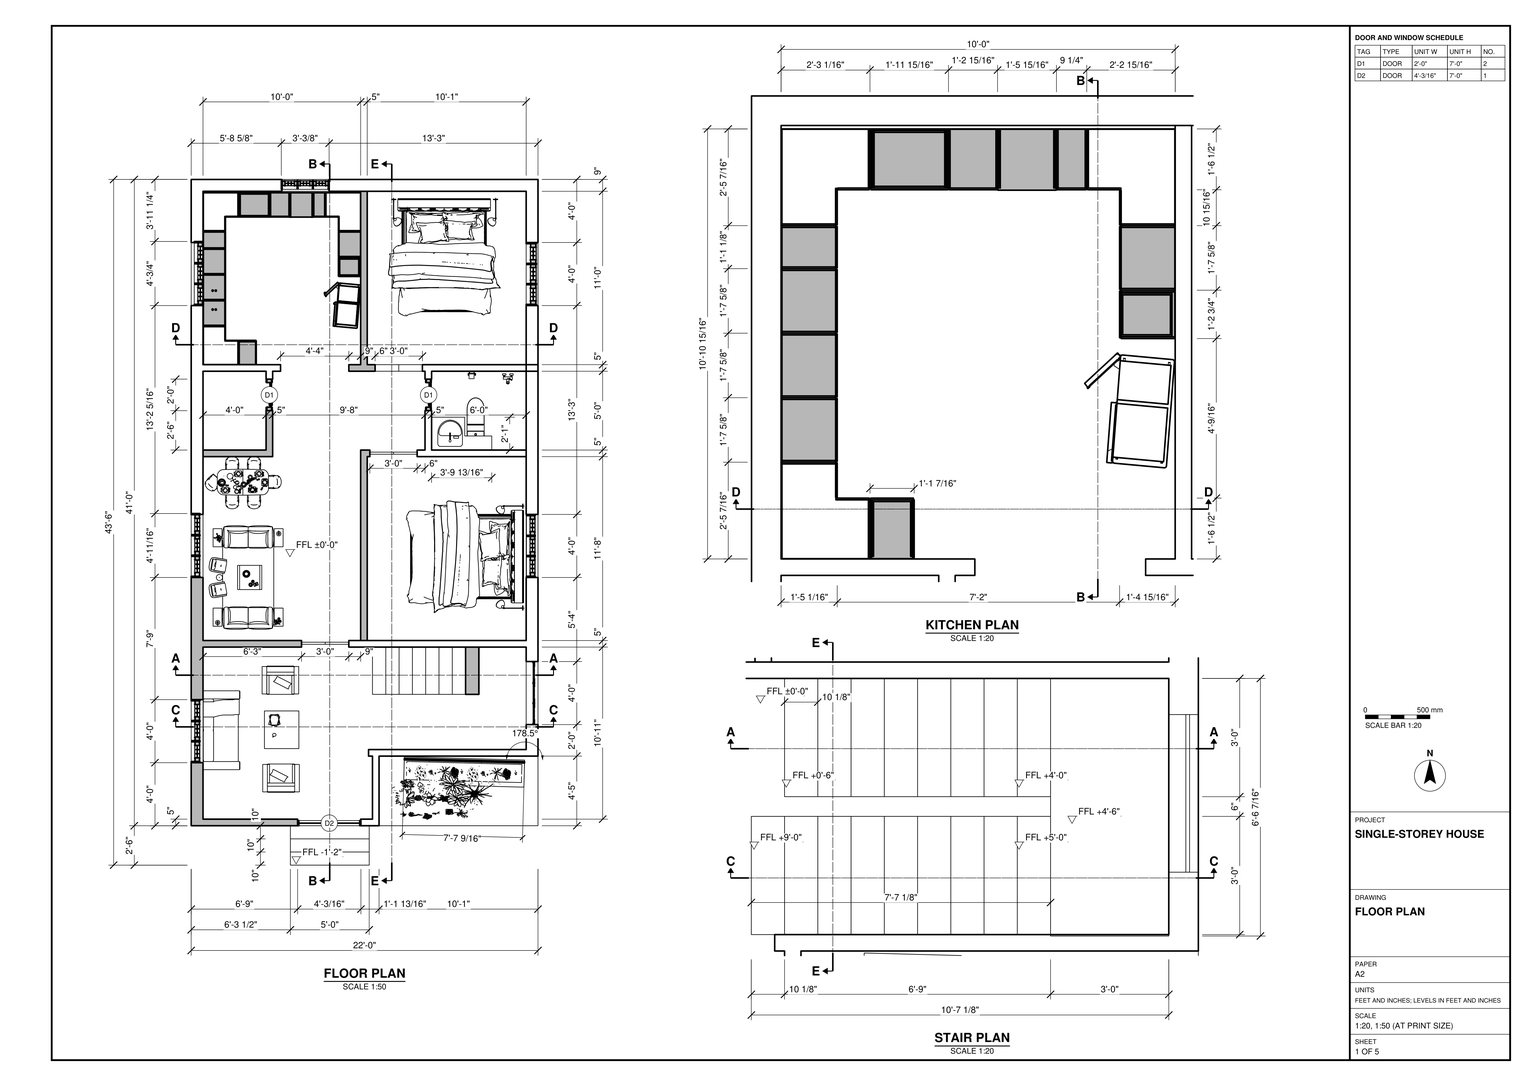
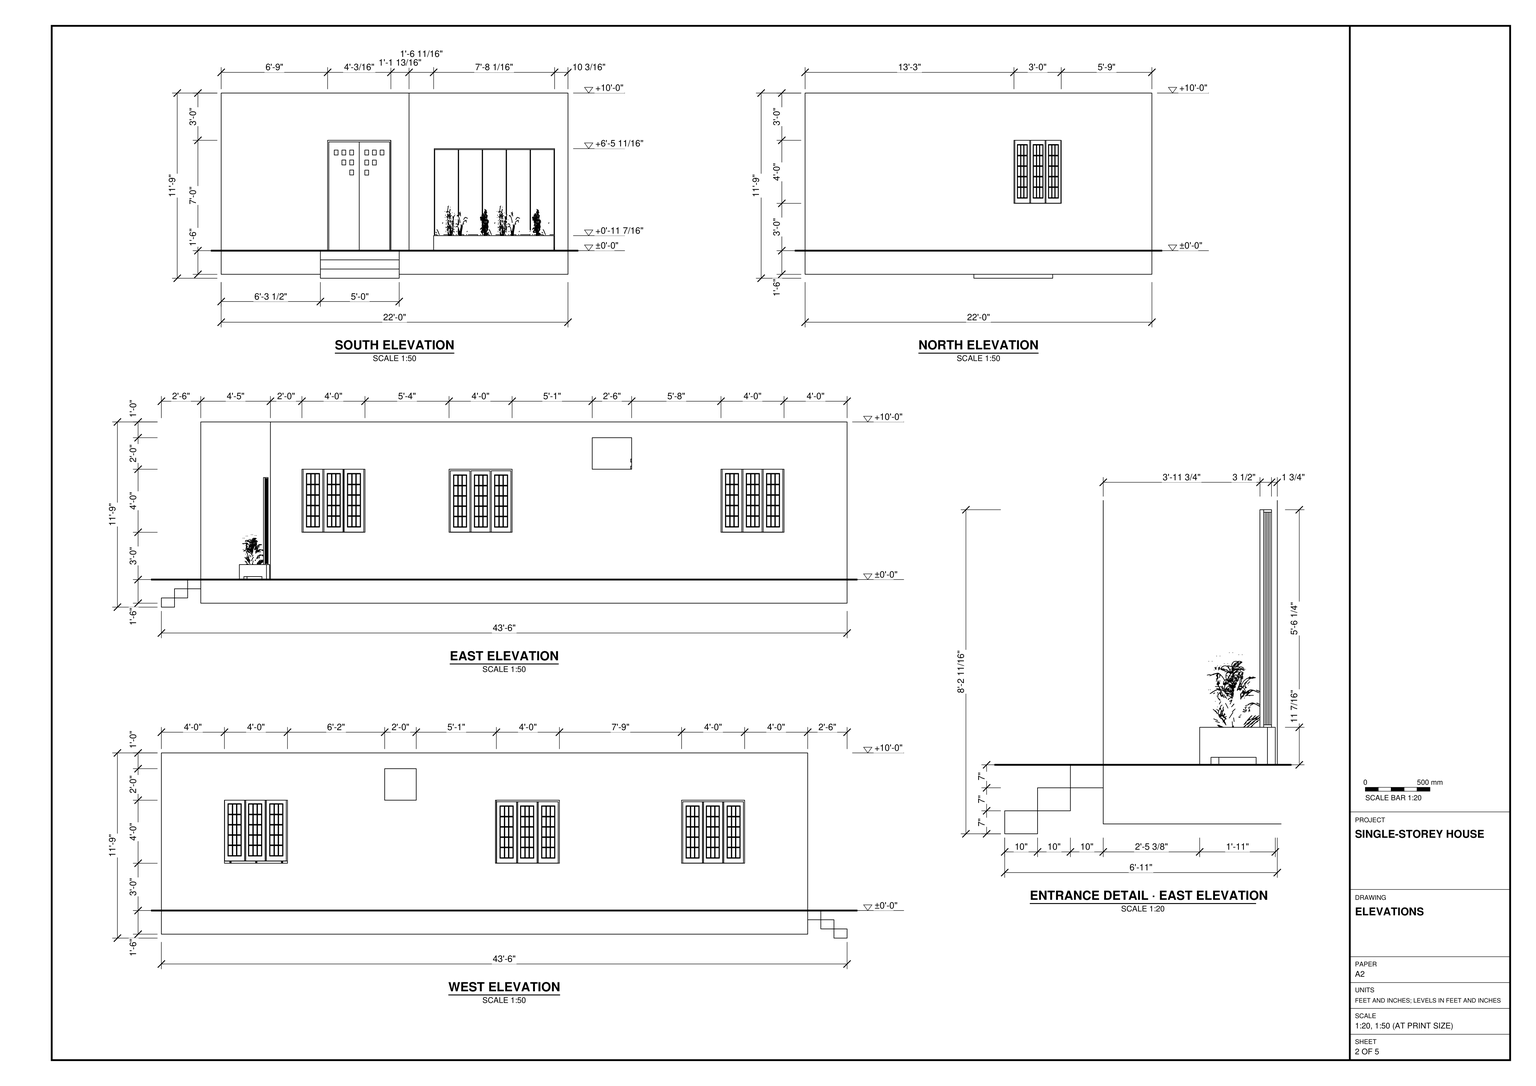
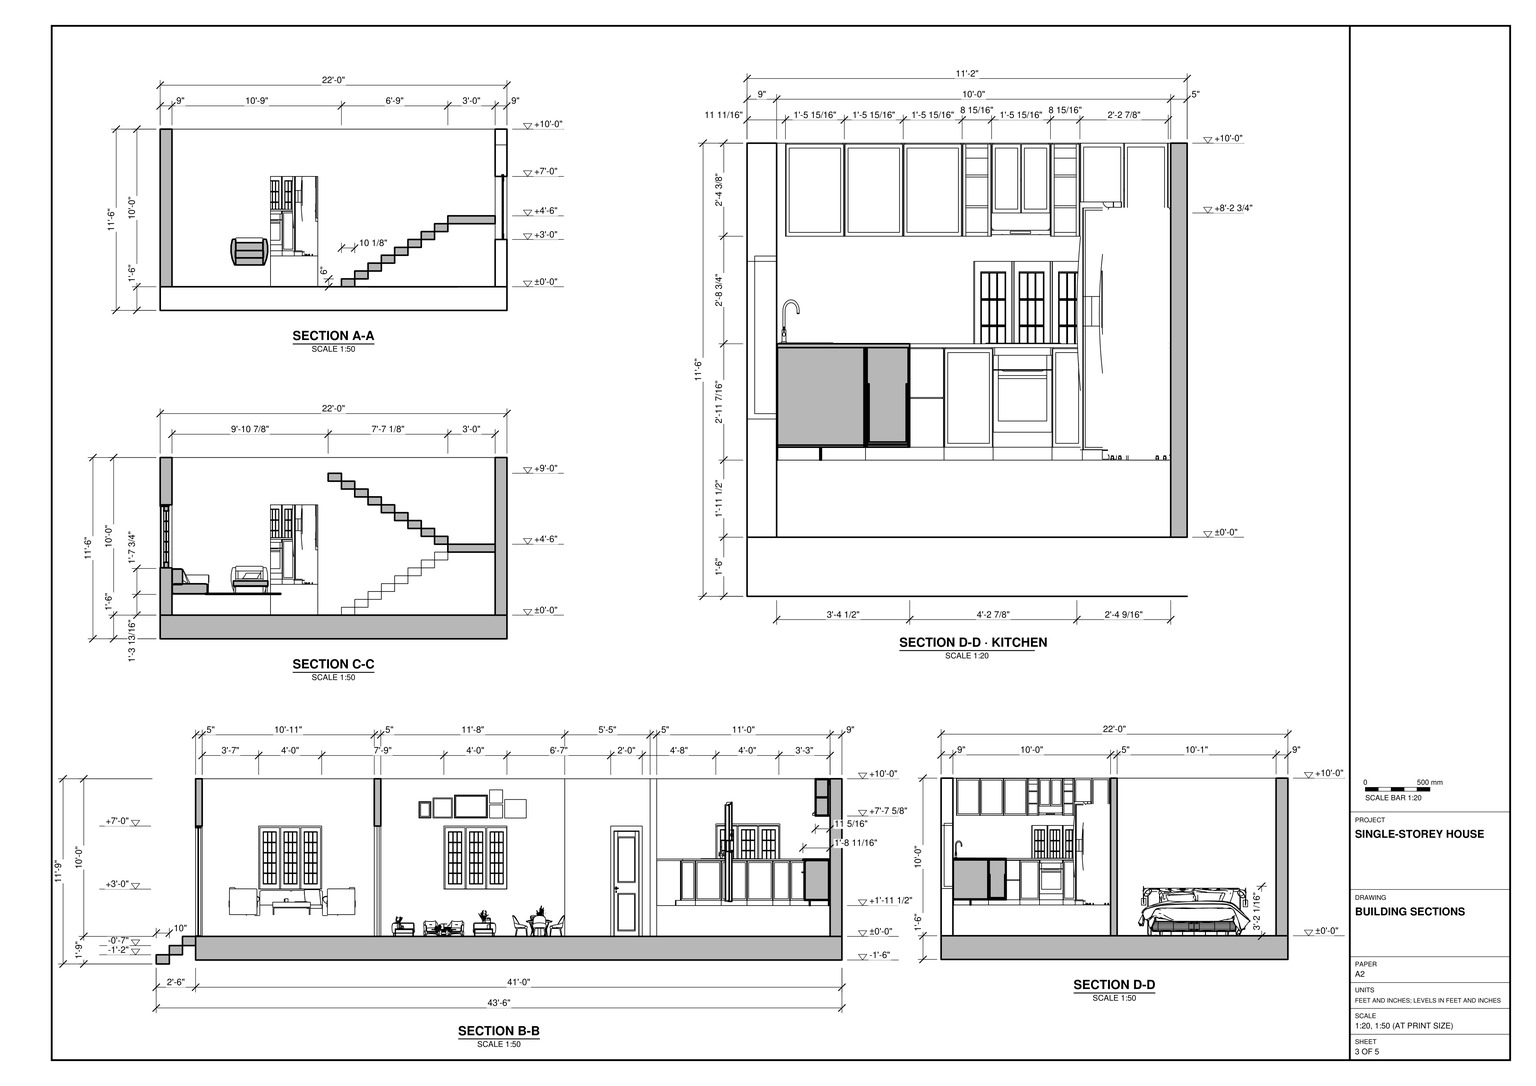
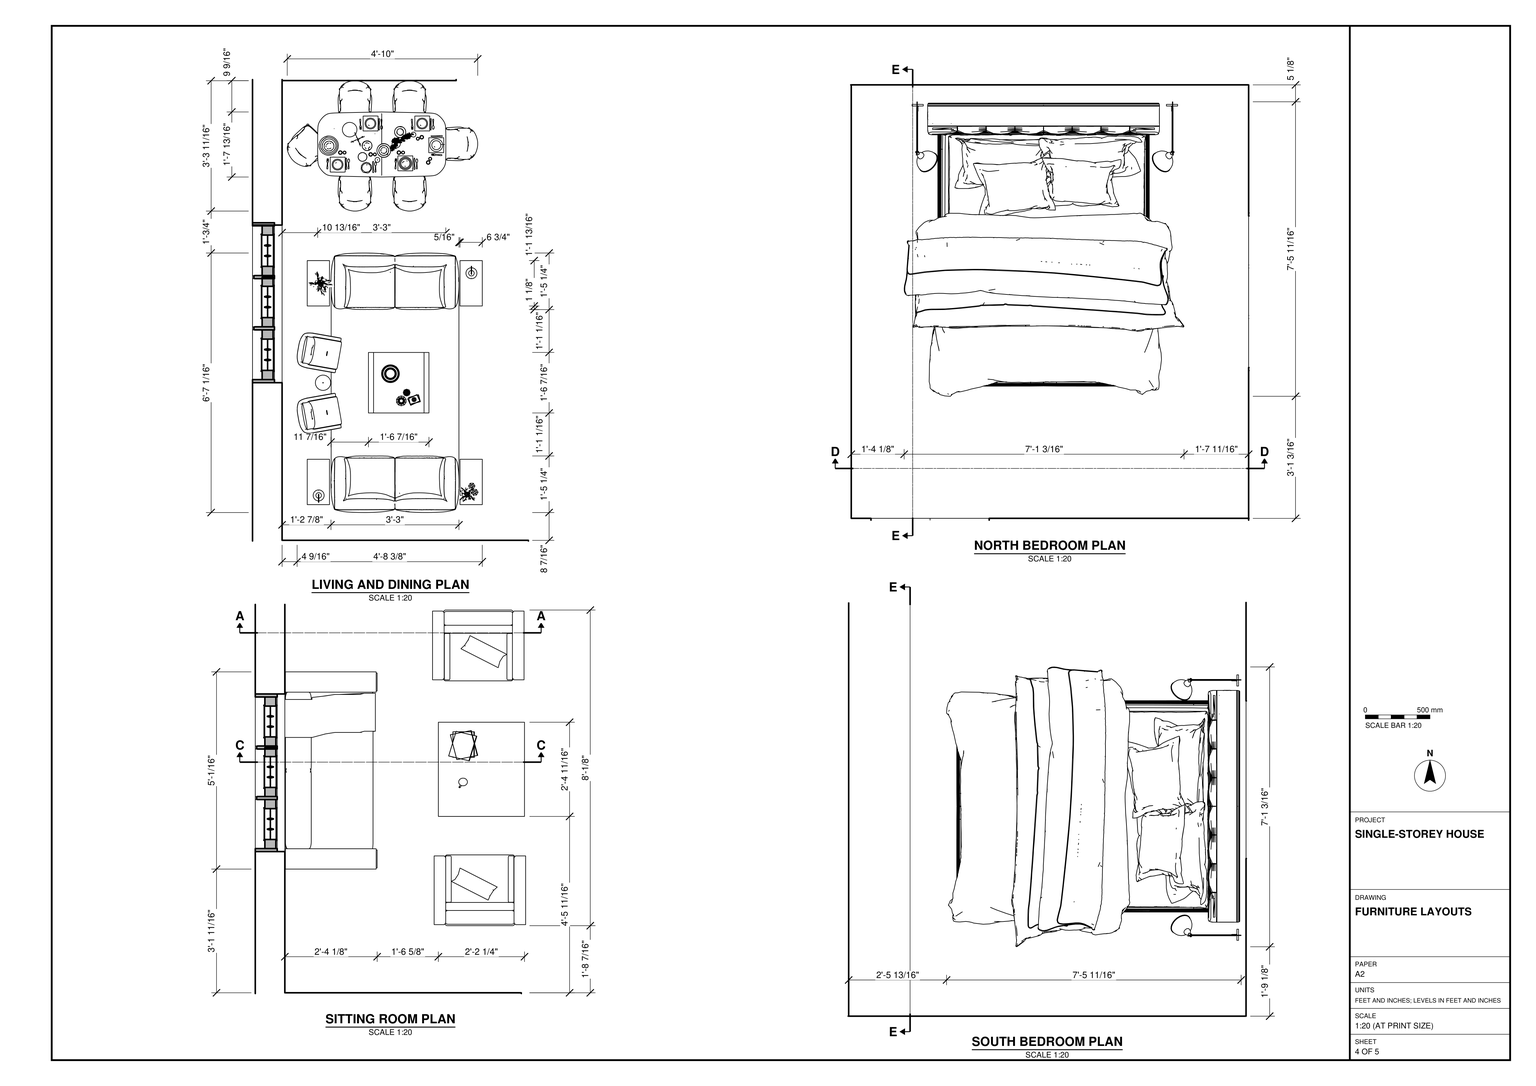
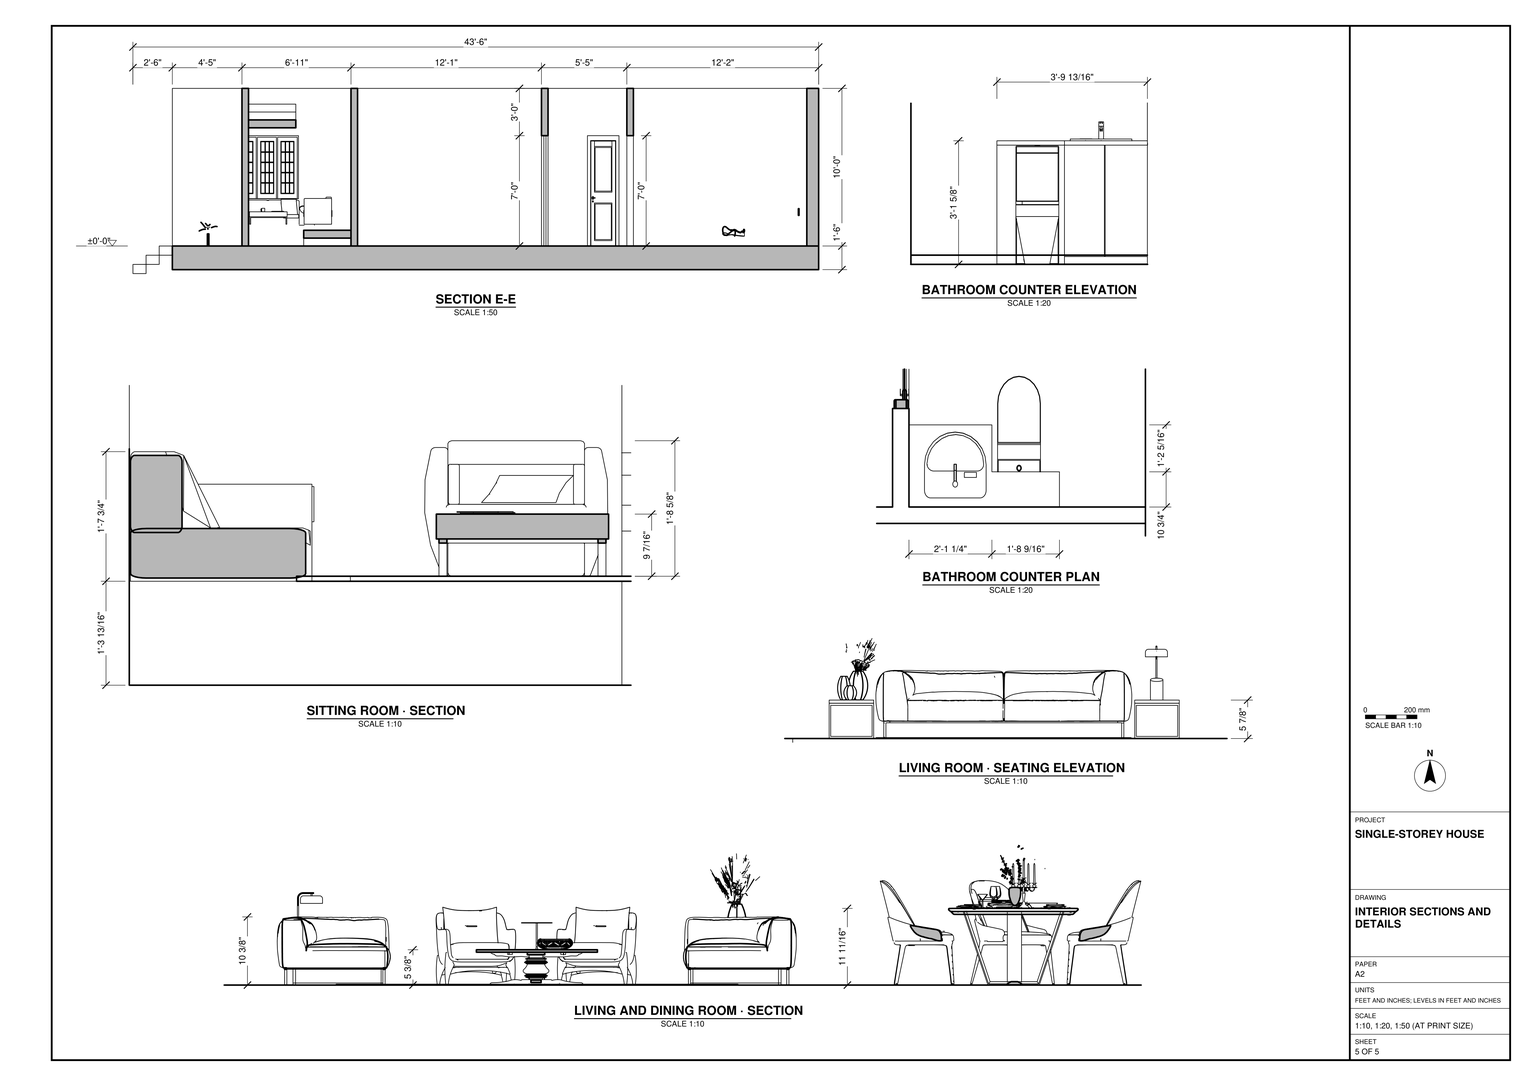
Build the single-storey house in SketchUp from task_files/diagram_01.pdf. Work in feet and inches. The overall size is 22'-0" wide by 43'-6" long, including the entrance steps, and 11'-9" high. Set the ground-floor finished level to ±0'-0". Model the raised floor slab and follow the plan for the thickness of each wall, distinguishing the 9" walls from the 5" walls.

At the south entrance, model the steps, paired doors and recessed planter with its screen. Place the front sitting area west of the return stair. Use the stair plan and sections to form the two opposing flights and their shared landing. Beyond the front sitting area, lay out the living and dining space on the west side, the two bedrooms on the east side and the small rooms off the central passage. Match the door and window positions to the plan and elevations.

Fit out the northwest kitchen with cabinet runs around the central workspace. Use the kitchen plan and section for the counters, cabinet divisions, upper units, sink and appliance positions. Match the footprints and orientations of the beds, seating and tables to the floor plan. Decor and loose items, including plants and appliances, may be any suitable library components.

Keep shell elements such as walls, slabs and any roof geometry separate as groups or components. Group each furniture or joinery piece separately and use components for repeated parts. Save one SketchUp model as output_files/furnished_single_storey_house_with_a_return_stair.skp.

# SketchUp Ruby script. Lengths in inches.
U = 1.inch
M = Sketchup.active_model
def pt(a) = Geom::Point3d.new(a.map { |v| v * U })
def face(e, loops, mat)
  f = e.add_face(loops[0].map { |a| pt(a) })
  loops[1..].each { |l| e.add_face(l.map { |a| pt(a) }).erase! }
  f.material = f.back_material = mat if mat
  f
end
# faces: each face lists its corners as indices into pts; further lists are holes
def faces(e, pts, list, mat = nil) = list.each { |f| face(e, (f[0].is_a?(Array) ? f : [f]).map { |l| l.map { |i| pts[i] } }, mat) }
# xy, xz, yz: faces in a plane at the given z, y or x. An outline is a flat list of corners, or four numbers for a rectangle; further outlines are holes
def ring(l) = l.size == 4 ? [[l[0], l[1]], [l[2], l[1]], [l[2], l[3]], [l[0], l[3]]] : l.each_slice(2).to_a
def flat(e, list, mat, &to3) = list.each { |f| face(e, (f[0].is_a?(Array) ? f : [f]).map { |l| ring(l).map { |u, v| to3.(u, v) } }, mat) }
def xy(e, z, list, mat = nil) = flat(e, list, mat) { |x, y| [x, y, z] }
def xz(e, y, list, mat = nil) = flat(e, list, mat) { |x, z| [x, y, z] }
def yz(e, x, list, mat = nil) = flat(e, list, mat) { |y, z| [x, y, z] }
def lines(e, pts, list) = list.each { |a, b| e.add_line(pt(pts[a]), pt(pts[b])) }
# prism: a flat outline (further loops are holes) pulled along v
def prism(e, loops, v, mat = nil)
  f = face(e, loops, mat); d = Geom::Vector3d.new(v.map { |x| x * U })
  f.pushpull(f.normal.samedirection?(d) ? d.length : -d.length)
end
def box(e, o, s, mat = nil) = prism(e, [[o, [o[0] + s[0], o[1], o[2]], [o[0] + s[0], o[1] + s[1], o[2]], [o[0], o[1] + s[1], o[2]]]], [0, 0, s[2]], mat)
def at(x, y, z, deg = 0) = Geom::Transformation.translation(pt([x, y, z])) * Geom::Transformation.rotation(ORIGIN, Z_AXIS, deg.degrees)
def axes(o, x, y, z) = Geom::Transformation.new([*x, 0, *y, 0, *z, 0, *pt(o).to_a, 1])
def part(name) = M.definitions.add(name)
# library, detail: a bought-in or finely detailed component or shape, given as its bounding box
def library(name, o, s) = part(name).tap { |d| box(d.entities, o, s) }
def detail(e, o, s) = box(e.add_group.entities, o, s)
def put(e, d, t, mat = nil) = e.add_instance(d, t).tap { |i| i.material = mat if mat }
def group(e, t, mat = nil) = e.add_group.tap { |g| g.transformation = t; g.material = mat if mat }.entities
root = M.entities
M.materials.add("1 (6)").color = [39, 39, 39]
M.materials.add("2").color = [201, 201, 201]
M.materials.add("3").color = [255, 255, 255]
M.materials.add("5").color = [30, 30, 30]
M.materials.add("6").color = [210, 193, 141]
M.materials.add("Material__1").color = [95, 70, 46]
M.materials.add("Sophie_Hair1").color = [198, 198, 198]
M.materials.add("Sophie_Hair2").color = [255, 255, 255]
M.materials.add("Steve_Hair1").color = [228, 228, 225]
M.materials.add("[0023_FireBrick]").color = [178, 34, 34]
M.materials.add("[0111_SlateGray]").color = [112, 128, 144]
M.materials.add("[0136_Charcoal]").color = [34, 34, 34]
M.materials.add("[Color M00]2").color = [255, 255, 255]
M.materials.add("[Color_008]1").color = [30, 30, 30]
M.materials.add("[Color_H05]").color = [204, 255, 255]
M.materials.add("[Marble Carrara Gold Floor Tile]").color = [225, 223, 217]
M.materials.add("[Pavers Modular Brick]").color = [175, 143, 129]
M.materials.add("[Square Glass Tile 01]").color = [123, 142, 151]
M.materials.add("[Stone Vein Gray]").color = [166, 165, 165]
M.materials.add("[Translucent Glass Gray]").color = [128, 128, 128]
M.materials.add("[Vegetation Grass Artificial]").color = [98, 140, 74]
M.materials.add("[White Square Tile]").color = [33, 33, 33]
M.materials.add("[sketch-stone]").color = [126, 99, 107]
M.materials.add("big").color = [85, 54, 44]
M.materials.add("cover").color = [255, 255, 255]
c1 = part("main door")
xy(c1.entities,0,[[0,0,3.9375,70.87]],"big")
xy(c1.entities,0.35,[[0,1.38,1.97,35.43],[1.97,1.38,3.9375,35.43],[0,35.43,1.97,69.49],[1.97,35.43,3.9375,69.49]],"big")
xy(c1.entities,93.11,[[0,1.38,1.97,35.43],[1.97,1.38,3.9375,35.43],[0,35.43,1.97,69.49],[1.97,35.43,3.9375,69.49]],"big")
xy(c1.entities,94.49,[[0,0,3.9375,70.87]],"big")
xz(c1.entities,0,[[0,0,3.9375,94.49]],"big")
xz(c1.entities,1.38,[[0,0.35,1.97,93.11],[1.97,0.35,3.9375,93.11]],"big")
xz(c1.entities,69.49,[[0,0.35,1.97,93.11],[1.97,0.35,3.9375,93.11]],"big")
xz(c1.entities,70.87,[[0,0,3.9375,94.49]],"big")
yz(c1.entities,0,[[[0,0,70.87,94.49],[1.38,0.35,69.49,93.11]]],"big")
yz(c1.entities,1.97,[[41.69,64.73,45.9,68.94],[24.84,64.85,29.05,69.06],[41.69,73.35,45.9,77.5625],[50.23,73.35,54.45,77.5625],[16.0625,73.43,20.27,77.64],
  [24.84,73.43,29.05,77.64],[7.48,81.93,11.69,86.14],[16.0625,81.93,20.27,86.14],[24.84,81.93,29.05,86.14],[41.69,81.93,45.9,86.14],
  [50.23,81.93,54.45,86.14],[58.82,81.93,63.03,86.14]],"[Color_H05]")
yz(c1.entities,1.97,[[[1.38,0.35,35.43,93.11],[24.84,81.93,29.05,86.14],[16.0625,81.93,20.27,86.14],[7.48,81.93,11.69,86.14],[24.84,73.43,29.05,77.64],[16.0625,73.43,20.27,77.64],[24.84,64.85,29.05,69.06]],[[35.43,0.35,69.49,93.11],[41.69,81.93,45.9,86.14],[50.23,81.93,54.45,86.14],[58.82,81.93,63.03,86.14],[50.23,73.35,54.45,77.5625],[41.69,73.35,45.9,77.5625],[41.69,64.73,45.9,68.94]]],"big")
yz(c1.entities,3.9375,[[[0,0,70.87,94.49],[1.38,0.35,69.49,93.11]]],"big")
c2 = part("d1")
xy(c2.entities,0,[[0,0,18,1.6],[18,0,36,1.6]],"[sketch-stone]")
xy(c2.entities,72,[[0,0,18,1.6],[18,0,36,1.6]],"[sketch-stone]")
yz(c2.entities,0,[[0,0,1.6,72]],"[sketch-stone]")
yz(c2.entities,36,[[0,0,1.6,72]],"[sketch-stone]")
c3 = library("Door C1",[0,0,0],[35.43,8.39,80.71])
c4 = library("The whole professional bed",[-16.91,-10.3,-0.31],[85.22,91.2,40.45])
c5 = library("Dining table set",[-3.55,-0.1,0],[135.47,90.42,53.12])
c6 = library("QUADRO-PAINTING",[182.91,225.91,15.99],[37.91,1.95,39.37])
c7 = part("Agrupar\#33")
xy(c7.entities,5.15,[[0,0,45.82,0.79]],"5")
xy(c7.entities,5.9375,[[0.79,0.39,45.03,0.55]],"3")
xy(c7.entities,5.9375,[[0.79,0.2,45.03,0.39],[0.79,0.55,45.03,0.79]],"5")
xy(c7.entities,7.12,[[1.97,0.39,43.85,0.47]],"3")
xy(c7.entities,35.04,[[1.97,0.39,43.85,0.47]],"3")
xy(c7.entities,36.22,[[0.79,0.39,45.03,0.55]],"3")
xy(c7.entities,36.22,[[0.79,0.2,45.03,0.39],[0.79,0.55,45.03,0.79]],"5")
xy(c7.entities,37.01,[[0,0,45.82,0.79]],"5")
xz(c7.entities,0.39,[[[0.79,5.9375,45.03,36.22],[1.97,7.12,43.85,35.04]]],"3")
xz(c7.entities,0.47,[[1.97,7.12,43.85,35.04]],"2")
xz(c7.entities,0.55,[[[0.79,5.9375,45.03,36.22],[1.97,7.12,43.85,35.04]]],"3")
xz(c7.entities,0.79,[[0,5.15,0,37.01,0.79,36.22,0.79,5.9375],[0,5.15,0.79,5.9375,45.03,5.9375,45.82,5.15],[45.82,5.15,45.03,5.9375,45.03,36.22,45.82,37.01],[0.79,36.22,0,37.01,45.82,37.01,45.03,36.22]],"5")
yz(c7.entities,0,[[0,5.15,0.79,37.01]],"5")
yz(c7.entities,0.79,[[0.39,5.9375,0.55,36.22]],"3")
yz(c7.entities,0.79,[[0.2,5.9375,0.39,36.22],[0.55,5.9375,0.79,36.22]],"5")
yz(c7.entities,1.97,[[0.39,7.12,0.47,35.04]],"3")
yz(c7.entities,43.85,[[0.39,7.12,0.47,35.04]],"3")
yz(c7.entities,45.03,[[0.39,5.9375,0.55,36.22]],"3")
yz(c7.entities,45.03,[[0.2,5.9375,0.39,36.22],[0.55,5.9375,0.79,36.22]],"5")
yz(c7.entities,45.82,[[0,5.15,0.79,37.01]],"5")
# 4 loose lines left out
p = [[0,0,5.15],[0.79,0.2,5.9375],[0.79,0.2,36.22],[0,0,37.01],[45.82,0,5.15],[45.03,0.2,5.9375],
  [0.79,0.79,5.9375],[0,0.79,5.15],[0.79,0.39,5.9375],[0.79,0.55,5.9375],[45.82,0,37.01],[45.03,0.2,36.22],
  [45.82,0.79,5.15],[45.03,0.79,5.9375],[45.03,0.55,5.9375],[45.03,0.39,5.9375],[0,0.79,37.01],[0.79,0.79,36.22],
  [0.79,0.55,36.22],[0.79,0.39,36.22],[45.03,0.79,36.22],[45.82,0.79,37.01],[45.03,0.39,36.22],[45.03,0.55,36.22]]
faces(c7.entities,p,[[0,1,2,3],[4,5,1,0],[4,10,11,5],[11,10,3,2]],"5")
faces(c7.entities,p,[[6,7,0,1,8,9],[12,13,14,15,5,4],[16,17,18,19,2,3],[20,21,10,11,22,23]])
c8 = part("Agrupar\#32")
xz(c8.entities,0,[[0,0,62.39,42.7]],"6")
c9 = part("Agrupar\#34")
put(c9.entities,c7,axes([0,0,-7.26],[1.41,0,0],[0,1.41,0],[0,0,1.41]))
put(c9.entities,c8,at(1.11,0.86,1.11))
c10 = part("quadro_morozini (1)")
put(c10.entities,c9,at(0,0,0))
c11 = part("TY004BG-B8686")
g1 = group(c11.entities,at(80,43.32,0))
xy(g1,0,[[0,0,33.86,2.36]],"Sophie_Hair1")
xy(g1,33.86,[[0,0,33.86,2.36]],"Sophie_Hair1")
xz(g1,0,[[0,0,33.86,33.86]])
xz(g1,2.36,[[0,0,33.86,33.86]],"Sophie_Hair1")
yz(g1,0,[[0,0,2.36,33.86]],"Sophie_Hair1")
yz(g1,33.86,[[0,0,2.36,33.86]],"Sophie_Hair1")
c12 = part("LN093B-967")
g2 = group(c12.entities,at(80,43.32,0))
xy(g2,0,[[0,0,31.89,2.36]],"Sophie_Hair2")
xy(g2,32.28,[[0,0,31.89,2.36]],"Sophie_Hair2")
xz(g2,0,[[0,0,31.89,32.28]])
xz(g2,2.36,[[0,0,31.89,32.28]],"Sophie_Hair2")
yz(g2,0,[[0,0,2.36,32.28]],"Sophie_Hair2")
yz(g2,31.89,[[0,0,2.36,32.28]],"Sophie_Hair2")
c13 = library("36",[-44.7,-74.43,-0.38],[89.21,170.96,60.16])
c14 = library("Areca palm plant",[0,0,0],[49.1,36.6,54.46])
c15 = part("W1")
xy(c15.entities,15,[[0,0,2,198]])
xy(c15.entities,102.0625,[[0,0,2,198]],"[Color M00]2")
xz(c15.entities,0,[[0,15,2,102.0625]],"[Color M00]2")
xz(c15.entities,198,[[0,15,2,102.0625]])
yz(c15.entities,0,[[0.84,16,39.43,101.0625],[40.28,16,78.87,101.0625],[79.71,16,118.3,101.0625],[119.14,16,157.73,101.0625],[158.58,16,197.16,101.0625]])
yz(c15.entities,0,[[[0,15,198,102.0625],[0.84,16,197.16,101.0625]],[39.43,16,40.28,101.0625],[78.87,16,79.71,101.0625],[118.3,16,119.14,101.0625],[157.73,16,158.58,101.0625]],"[Color M00]2")
yz(c15.entities,2,[[0.84,16,39.43,101.0625],[40.28,16,78.87,101.0625],[79.71,16,118.3,101.0625],[119.14,16,157.73,101.0625],[158.58,16,197.16,101.0625]])
yz(c15.entities,2,[[[0,15,198,102.0625],[0.84,16,197.16,101.0625]],[39.43,16,40.28,101.0625],[78.87,16,79.71,101.0625],[118.3,16,119.14,101.0625],[157.73,16,158.58,101.0625]],"[Color M00]2")
c16 = library("Group\#220",[-84.69,-90.07,-0.36],[176.51,175.13,171.4])
c17 = library("Group20\#1",[-20.81,-17.08,3.79],[39.86,39.43,37.51])
c18 = library("Group\#221",[-7.34,-1.2,0],[38.67,35.81,49.04])
c19 = library("Group38\#2",[14.01,28.44,-23.43],[18.58,18.32,38.89])
c20 = part("PLANTS")
put(c20.entities,c14,axes([38.49,169.84,6.02],[0.45017,-0.56191,0],[0.66137,0.52986,0],[0,0,0.72]))
put(c20.entities,c14,axes([38.49,68.02,6.02],[0.45017,-0.56191,0],[0.66137,0.52986,0],[0,0,0.72]))
put(c20.entities,c15,axes([76.68,11.43,-0.0625],[1,0,0],[0,1.18586,0],[0,0,1]),"[Translucent Glass Gray]")
put(c20.entities,c16,axes([59.61,184.54,5.99],[-0.04961,-0.08593,0],[0.08593,-0.04961,0],[0,0,0.10522]))
put(c20.entities,c16,axes([59.61,204.61,5.99],[-0.04961,-0.08593,0],[0.08593,-0.04961,0],[0,0,0.10522]))
put(c20.entities,c16,axes([59.61,157.29,5.99],[-0.04961,-0.08593,0],[0.08593,-0.04961,0],[0,0,0.10522]))
put(c20.entities,c17,axes([63.65,91.4,4.71],[0,0.85,0],[-0.85,0,0],[0,0,0.85]))
put(c20.entities,c18,axes([69.62,101.34,7.93],[0,0.79,0],[-0.79,0,0],[0,0,0.79]))
put(c20.entities,c19,axes([40.58,10.27,28.11],[0.8848,0,0],[0,0.94674,0],[0,0,0.85826]))
put(c20.entities,c16,axes([59.61,55.48,5.99],[-0.04961,-0.08593,0],[0.08593,-0.04961,0],[0,0,0.10522]))
put(c20.entities,c16,axes([59.61,82.73,5.99],[-0.04961,-0.08593,0],[0.08593,-0.04961,0],[0,0,0.10522]))
put(c20.entities,c16,axes([61.875,132.66,6.01],[-0.08133,-0.14087,0],[0.14087,-0.08133,0],[0,0,0.1725]))
put(c20.entities,c16,axes([59.61,102.79,5.99],[-0.04961,-0.08593,0],[0.08593,-0.04961,0],[0,0,0.10522]))
put(c20.entities,c16,axes([61.875,27.22,6.01],[-0.08133,-0.14087,0],[0.14087,-0.08133,0],[0,0,0.1725]))
put(c20.entities,c16,axes([61.875,234.47,6.01],[-0.08133,-0.14087,0],[0.14087,-0.08133,0],[0,0,0.1725]))
put(c20.entities,c18,axes([69.62,203.15,7.93],[0,0.79,0],[-0.79,0,0],[0,0,0.79]))
put(c20.entities,c17,axes([63.65,193.21,4.71],[0,0.85,0],[-0.85,0,0],[0,0,0.85]))
put(c20.entities,c19,axes([40.58,112.08,28.11],[0.8848,0,0],[0,0.94674,0],[0,0,0.85826]))
g3 = group(c20.entities,at(44.68,11.43,-0.0625))
xy(g3,0,[[0,0,6,234.8],[30,0,36,234.8]])
xy(g3,3,[[6,0,30,234.8]])
xy(g3,7,[[6,5,30,229.8]],"Material__1")
xy(g3,15,[[[0,0,36,234.8],[6,5,30,229.8]]])
xz(g3,0,[[0,0,6,0,6,3,30,3,30,0,36,0,36,15,0,15]])
xz(g3,5,[[6,7,30,15]])
xz(g3,229.8,[[6,7,30,15]])
xz(g3,234.8,[[0,0,0,15,36,15,36,0,30,0,30,3,6,3,6,0]])
yz(g3,0,[[0,0,234.8,15]])
yz(g3,6,[[0,0,234.8,3],[5,7,229.8,15]])
yz(g3,30,[[0,0,234.8,3],[5,7,229.8,15]])
yz(g3,36,[[0,0,234.8,15]])
c21 = part("Group\#5")
box(c21.entities,[0,0,0],[10.125,36,6])
c22 = part("Group\#7")
box(c22.entities,[0,0,0],[60,10,7])
c23 = library("Group\#61",[0,0,0],[50.37,77,85.15])
c24 = library("Group\#67",[0.125,0,0],[4,104,82])
c25 = library("Group\#99",[0,0,0],[158.07,157.48,96.53])
c26 = part("Группа\#47")
xy(c26.entities,0,[[0,0,23.31,20.55]],"[0136_Charcoal]")
xy(c26.entities,0.2,[[0.36,0.64,22.93,20.59]],"[White Square Tile]")
p = [[0.36,20.13,0.2],[0.36,0.64,0.2],[0,0,0],[0,20.55,0],[0.36,20.59,0.2],[22.93,0.64,0.2],
  [23.31,0,0],[23.31,20.55,0],[22.93,20.13,0.2],[22.93,20.5625,0.2],[22.93,20.59,0.2]]
faces(c26.entities,p,[[0,1,2,3,4],[1,5,6,2],[7,6,5,8,9,10],[3,7,10,4]],"[0136_Charcoal]")
c27 = library("Agrupar\#2",[0,-7.38,0],[12.4,73.82,70.87])
c28 = library("Group\#182",[0,0,0],[82.79,96.12,21.4])
c29 = part("Agrupar\#36")
prism(c29.entities,[[[9.45,12.875,-0.1],[9.45,0,-0.1],[0,0,-0.1],[0,12.875,-0.1]],[[8.86,0.59,-0.1],[8.86,12.28,-0.1],[0.59,12.28,-0.1],[0.59,0.59,-0.1]]],[0,0,0.39],"[Color_008]1")
c30 = part("Agrupar\#35")
xy(c30.entities,0,[[0,0,8.27,11.69]])
xy(c30.entities,0.1,[[0.79,0.79,7.48,10.91]],"1 (6)")
xy(c30.entities,0.1,[[[0,0,8.27,11.69],[0.79,0.79,7.48,10.91]]],"cover")
xz(c30.entities,0,[[0,0,8.27,0.1]])
xz(c30.entities,11.69,[[0,0,8.27,0.1]])
yz(c30.entities,0,[[0,0,11.69,0.1]])
yz(c30.entities,8.27,[[0,0,11.69,0.1]])
c31 = part("Agrupar\#37")
put(c31.entities,c29,at(0,0,0.1))
put(c31.entities,c30,at(0.59,0.59,0.1))
c32 = library("Group\#183",[-0.62,0,0],[57,79.03,20.625])
xy(root,-18,[[0,30,264,522]])
xy(root,0,[[0,30,143,30,143,83,264,83,264,522,0,522]],"[Marble Carrara Gold Floor Tile]")
xy(root,0,[[143,30,264,83]],"[Vegetation Grass Artificial]")
xz(root,30,[[0,-18,264,0]])
xz(root,522,[[0,-18,264,0]])
yz(root,0,[[30,-18,522,0]])
yz(root,264,[[30,-18,522,0]])
put(root,c1,axes([81,33.9375,0],[0,-1,0],[0.68,0,0],[0,0,0.889]))
put(root,c2,axes([140,376,0],[1,0,0],[0,3.125,0],[0,0,1.16667]))
put(root,c2,axes([136,312.83,0],[1,0,0],[0,1,0],[0,0,1.16667]))
put(root,c2,axes([84,168.125,0],[1,0,0],[0,1,0],[0,0,1.16667]))
put(root,c3,axes([178.5,370,0],[0,-0.67733,0],[0.53605,0,0],[0,0,1.04078]))
put(root,c3,axes([57.0625,370,0],[0,-0.67733,0],[0.58819,0,0],[0,0,1.04078]))
put(root,c4,at(167.02,428.46,0))
put(root,c4,at(174.1,260.43,0.31,-90))
put(root,c5,axes([10.5625,271.26,0],[0.44,0,0],[0,0.44,0],[0,0,0.44]))
put(root,c6,axes([100.93,139.36,83.86],[0,0.39,0],[-0.39,0,0],[0,0,0.39]))
put(root,c10,axes([12.83,227.01,90.11],[0,0.39,0],[-0.39,0,0],[0,0,0.39]))
put(root,c11,axes([28.04,230.14,90.11],[0,0.29504,0],[-0.34961,0,0],[0,0,0.29504]))
put(root,c12,axes([28.04,228.68,101.46],[0,0.31325,0],[-0.34961,0,0],[0,0,0.31239]))
put(root,c13,axes([181.73,52.19,0.15],[0,-0.39161,0],[0.51415,0,0],[0,0,0.39161]))
put(root,c20,axes([257.04,33.64,0.05],[0.01501,0.5731,0],[-0.38987,0.01021,0],[0,0,0.76112]),"[Vegetation Grass Artificial]")
g4 = group(root,at(0,30,0))
xy(g4,0,[[0,0,0,492,264,492,264,351,255,351,255,483,9,483,9,351,68,351,68,346,62,346,62,340,57,340,57,346,9,346,9,141,84,141,84,136,9,136,9,5,81,5,81,0],[129,0,129,5,138,5,138,53,135,53,135,58,255,58,255,136,120,136,120,141,255,141,255,346,264,346,264,53,143,53,143,0],[129,141,129,286,136,286,136,281,134,281,134,141],[9,281,62,286],[172,281,172,286,178,286,178,316,183,316,183,286,255,286,255,281],
  [57,286,62,316],[178,340,178,346,176,346,176,351,255,351,255,346,183,346,183,340],[120,346,120,351,129,351,129,483,134,483,134,351,140,351,140,346]])
xy(g4,2.8125,[[183,286,255,346]],"[Square Glass Tile 01]")
xy(g4,36,[[0,48,9,96],[255,77,264,125],[0,189,9,237],[255,189,264,237],[0,396,9,444],
  [255,396,264,444],[69,483,105,492]])
xy(g4,84,[[81,0,129,5],[0,48,9,96],[255,77,264,125],[84,136,120,141],[0,189,9,237],
  [255,189,264,237],[136,281,172,286],[0,298,9,322],[255,298,264,328],[57,316,62,340],
  [178,316,183,340],[140,346,176,351],[0,396,9,444],[255,396,264,444],[69,483,105,492]])
xy(g4,108,[[0,298,9,322],[255,298,264,328]])
xy(g4,120,[[0,0,143,0,143,53,264,53,264,346,255,346,255,141,120,141,120,136,255,136,255,58,135,58,135,53,138,53,138,5,9,5,9,136,120,136,120,141,9,141,9,346,57,346,57,340,62,340,62,346,68,346,68,351,9,351,9,483,255,483,255,351,264,351,264,492,0,492],[129,141,134,141,134,281,172,281,172,286,129,286],[9,281,62,286],[172,281,255,281,255,286,183,286,183,340,178,340,178,286,172,286],[57,286,62,340],
  [178,340,183,340,183,346,255,346,255,351,176,351,176,346,178,346],[120,346,176,346,176,351,134,351,134,483,129,483,129,351,120,351],[255,346,264,351]])
xz(g4,0,[[0,0,81,0,81,84,129,84,129,0,143,0,143,120,0,120]],"[0023_FireBrick]")
xz(g4,5,[[9,0,9,120,129,120,129,84,81,84,81,0],[129,0,138,120]])
xz(g4,48,[[0,36,9,84]])
xz(g4,53,[[135,0,138,120]])
xz(g4,53,[[143,0,264,120]],"[Pavers Modular Brick]")
xz(g4,58,[[135,0,255,120]])
xz(g4,77,[[255,36,264,84]])
xz(g4,96,[[0,36,9,84]])
xz(g4,125,[[255,36,264,84]])
xz(g4,136,[[9,0,84,0,84,84,120,84,120,120,9,120],[120,0,255,120]])
xz(g4,141,[[9,0,9,120,120,120,120,84,84,84,84,0],[120,0,129,120],[129,0,134,120],[134,0,255,120]])
xz(g4,189,[[0,36,9,84],[255,36,264,84]])
xz(g4,237,[[0,36,9,84],[255,36,264,84]])
xz(g4,281,[[9,0,62,120],[134,0,136,0,136,84,172,84,172,120,134,120],[172,0,255,120]])
xz(g4,286,[[9,0,57,120],[129,0,129,120,172,120,172,84,136,84,136,0],[172,0,178,120],[183,0,255,2.8125]])
xz(g4,286,[[183,2.8125,255,120]],"[Square Glass Tile 01]")
xz(g4,298,[[0,84,9,108],[255,84,264,108]])
xz(g4,316,[[57,0,62,84],[178,0,183,84]])
xz(g4,322,[[0,84,9,108]])
xz(g4,328,[[255,84,264,108]])
xz(g4,340,[[57,0,62,84],[178,0,183,84]])
xz(g4,346,[[9,0,57,120],[62,0,68,120],[120,0,140,0,140,84,176,84,176,120,120,120],[176,0,178,120],[183,0,255,2.8125],
  [255,0,264,120]])
xz(g4,346,[[183,2.8125,255,120]],"[Square Glass Tile 01]")
xz(g4,351,[[9,0,68,120],[120,0,129,120],[134,0,134,120,176,120,176,84,140,84,140,0],[176,0,255,120],[255,0,264,120]])
xz(g4,396,[[0,36,9,84],[255,36,264,84]])
xz(g4,444,[[0,36,9,84],[255,36,264,84]])
xz(g4,483,[[[9,0,129,120],[69,36,105,84]],[129,0,134,120],[134,0,255,120]])
xz(g4,492,[[[0,0,264,120],[69,36,105,84]]],"[0023_FireBrick]")
yz(g4,0,[[[0,0,492,120],[48,36,96,84],[189,36,237,84],[396,36,444,84],[298,84,322,108]]],"[0023_FireBrick]")
yz(g4,9,[[[5,0,136,120],[48,36,96,84]],[[141,0,281,120],[189,36,237,84]],[281,0,286,120],[[286,0,346,120],[298,84,322,108]],[[351,0,483,120],[396,36,444,84]]])
yz(g4,57,[[286,0,286,120,340,120,340,84,316,84,316,0],[340,0,346,120]])
yz(g4,62,[[281,0,316,0,316,84,340,84,340,120,281,120],[340,0,346,120]])
yz(g4,68,[[346,0,351,120]])
yz(g4,69,[[483,36,492,84]])
yz(g4,81,[[0,0,5,84]])
yz(g4,84,[[136,0,141,84]])
yz(g4,105,[[483,36,492,84]])
yz(g4,120,[[136,0,141,84],[346,0,351,120]])
yz(g4,129,[[0,0,5,84],[141,0,286,120],[351,0,483,120]])
yz(g4,134,[[141,0,281,120],[351,0,483,120]])
yz(g4,135,[[53,0,58,120]])
yz(g4,136,[[281,0,286,84]])
yz(g4,138,[[5,0,53,120]])
yz(g4,140,[[346,0,351,84]])
yz(g4,143,[[0,0,53,120]],"[0111_SlateGray]")
yz(g4,172,[[281,0,286,84]])
yz(g4,176,[[346,0,351,84]])
yz(g4,178,[[286,0,286,120,340,120,340,84,316,84,316,0],[340,0,346,120]])
yz(g4,183,[[286,0,316,2.8125],[340,0,346,2.8125]])
yz(g4,183,[[286,2.8125,316,2.8125,316,84,340,84,340,120,286,120],[340,2.8125,346,120]],"[Square Glass Tile 01]")
yz(g4,255,[[[58,0,136,120],[77,36,125,84]],[[141,0,281,120],[189,36,237,84]],[281,0,286,120],[286,0,346,2.8125],[346,0,351,120],
  [[351,0,483,120],[396,36,444,84]]])
yz(g4,255,[[[286,2.8125,346,120],[298,84,328,108]]],"[Square Glass Tile 01]")
yz(g4,264,[[[53,0,346,120],[189,36,237,84],[77,36,125,84],[298,84,328,108]],[346,0,351,120],[[351,0,492,120],[396,36,444,84]]],"[0023_FireBrick]")
# 2 loose lines left out
g5 = group(root,at(138,88,0))
p = [[70.875,42,0],[70.875,78,0],[60.75,42,0],[0,36,0],[10.125,36,0],[70.875,0,0],
  [70.875,36,0],[81,42,0],[81,78,0],[81,36,0],[50.625,42,0],[50.625,78,0],
  [30.375,42,0],[30.375,78,0],[20.25,42,0],[40.5,42,0],[81,0,0],[10.125,42,0],
  [60.75,78,0],[20.25,78,0],[10.125,78,0],[0,42,0],[40.5,78,0],[0,78,0],
  [10.125,0,0],[30.375,0,0],[30.375,36,0],[20.25,36,0],[40.5,0,0],[40.5,36,0],
  [0,0,0],[60.75,36,0],[50.625,0,0],[50.625,36,0],[60.75,0,0],[20.25,0,0]]
lines(g5,p,[[0,1],[0,2],[3,4],[5,6],[7,8],[9,7],[10,11],[12,13],[2,10],[12,14],[15,12],[16,9],
  [10,15],[14,17],[6,9],[2,18],[14,19],[17,20],[17,21],[15,22],[21,23],[24,4],[25,26],[4,27],
  [28,29],[26,29],[30,3],[7,0],[31,6],[21,3],[32,33],[34,31],[33,31],[29,33],[35,27],[27,26]])
put(root,c21,at(138,130,0),"[Stone Vein Gray]")
put(root,c21,at(148.125,130,6),"[Stone Vein Gray]")
put(root,c21,at(158.25,130,12),"[Stone Vein Gray]")
put(root,c21,at(168.375,130,18),"[Stone Vein Gray]")
put(root,c21,at(178.5,130,24),"[Stone Vein Gray]")
put(root,c21,at(188.625,130,30),"[Stone Vein Gray]")
put(root,c21,at(198.75,130,36),"[Stone Vein Gray]")
put(root,c21,at(208.875,130,42),"[Stone Vein Gray]")
g6 = group(root,at(219,130,48),"[Stone Vein Gray]")
box(g6,[0,-42.4375,0],[36,78.4375,6])
put(root,c21,at(208.875,88,54),"[Stone Vein Gray]")
put(root,c21,at(198.75,88,60),"[Stone Vein Gray]")
put(root,c21,at(188.625,88,66),"[Stone Vein Gray]")
put(root,c21,at(178.5,88,72),"[Stone Vein Gray]")
put(root,c21,at(168.375,88,78),"[Stone Vein Gray]")
put(root,c21,at(158.25,88,84),"[Stone Vein Gray]")
put(root,c21,at(148.125,88,90),"[Stone Vein Gray]")
put(root,c21,at(138,88,96),"[Stone Vein Gray]")
g7 = group(root,at(127.875,88,102),"[Stone Vein Gray]")
box(g7,[0,0,0],[10.125,36,6])
put(root,c22,at(75.51,20,-7),"[Stone Vein Gray]")
put(root,c22,at(75.51,10,-14),"[Stone Vein Gray]")
put(root,c22,at(75.51,0,-21),"[Stone Vein Gray]")
put(root,c23,axes([183,376,0],[0,-1.19125,0],[0.93506,0,0],[0,0,1.1214]))
put(root,c24,axes([105,514.25,36],[0,1.67,0],[-0.35,0,0],[0,0,0.6]))
put(root,c24,axes([-0.21,78,36],[1.67,0,0],[0,0.46154,0],[0,0,0.58537]))
put(root,c24,axes([-0.21,219,36],[1.67,0,0],[0,0.46827,0],[0,0,0.58537]))
put(root,c24,axes([2.11,426,37.625],[1.67,0,0],[0,0.469,0],[0,0,0.58537]))
put(root,c24,axes([254.76,426,36],[1.9539,0,0],[0,0.46154,0],[0,0,0.6]))
put(root,c24,axes([255,219,36],[1.67,0,0],[0,0.46154,0],[0,0,0.58537]))
put(root,c24,axes([260.16,107,36],[0.2839,0,0],[0,0.46154,0],[0,0,0.6]))
put(root,c25,axes([9,381,23.47],[0.75918,0,0],[0,0.8316,0],[0,0,1]),"Steve_Hair1")
put(root,c26,at(72.43,492.32,58.91))
put(root,c27,axes([128.31,267.06,49.7],[-0.832,0,0],[0,-0.5876,0],[0,0,0.65]))
put(root,c28,at(9,55.4375,15.83))
g8 = group(root,at(12.71,265.27,90.11))
box(g8,[-0.83,0,0],[0.83,16.43,14.1])
put(root,c31,axes([12.07,199.95,90.11],[0,0.975,0],[0,0,0.975],[2.89182,0,0]))
put(root,c32,at(13.58,179.46,0))
